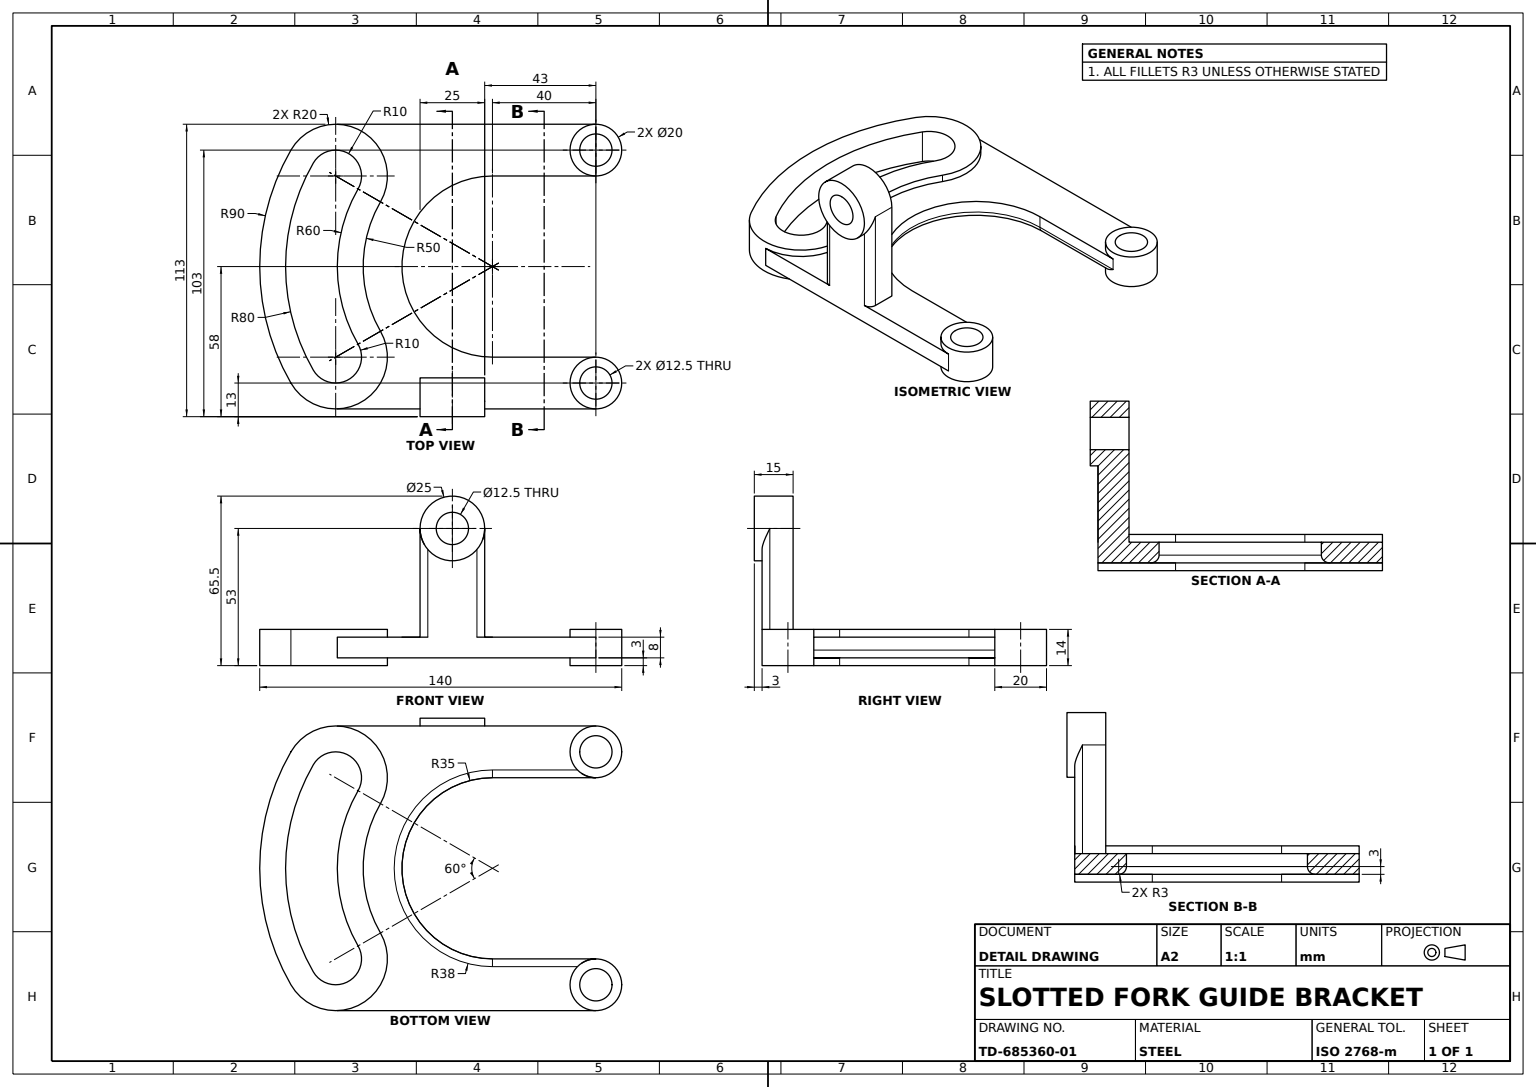
ISO-10303-21;
HEADER;
FILE_DESCRIPTION((''),'2;1');
FILE_NAME('','',(''),(''),'','','');
FILE_SCHEMA(('AUTOMOTIVE_DESIGN'));
ENDSEC;
DATA;
#1=APPLICATION_CONTEXT('');
#2=PRODUCT_CONTEXT('',#1,'mechanical');
#3=PRODUCT('','','',(#2));
#4=PRODUCT_DEFINITION_FORMATION('','',#3);
#5=PRODUCT_DEFINITION_CONTEXT('',#1,'design');
#6=PRODUCT_DEFINITION('','',#4,#5);
#7=PRODUCT_DEFINITION_SHAPE('','',#6);
#8=(LENGTH_UNIT()NAMED_UNIT(*)SI_UNIT(.MILLI.,.METRE.));
#9=(NAMED_UNIT(*)PLANE_ANGLE_UNIT()SI_UNIT($,.RADIAN.));
#10=(NAMED_UNIT(*)SI_UNIT($,.STERADIAN.)SOLID_ANGLE_UNIT());
#11=UNCERTAINTY_MEASURE_WITH_UNIT(LENGTH_MEASURE(0.005),#8,'distance_accuracy_value','');
#12=(GEOMETRIC_REPRESENTATION_CONTEXT(3)GLOBAL_UNCERTAINTY_ASSIGNED_CONTEXT((#11))GLOBAL_UNIT_ASSIGNED_CONTEXT((#8,#9,#10))REPRESENTATION_CONTEXT('',''));
#13=CARTESIAN_POINT('',(-77.942286,-45.,7.));
#14=VERTEX_POINT('',#13);
#15=CARTESIAN_POINT('',(-77.942286,-45.,-7.));
#16=VERTEX_POINT('',#15);
#17=DIRECTION('',(0.,0.,-1.));
#18=VECTOR('',#17,1000.);
#19=LINE('',#13,#18);
#20=EDGE_CURVE('',#14,#16,#19,.T.);
#21=ORIENTED_EDGE('',*,*,#20,.T.);
#22=CARTESIAN_POINT('',(-43.30127,-25.,-7.));
#23=VERTEX_POINT('',#22);
#24=CARTESIAN_POINT('',(-60.621778,-35.,-7.));
#25=DIRECTION('',(0.,0.,1.));
#26=DIRECTION('',(1.,0.,0.));
#27=AXIS2_PLACEMENT_3D('',#24,#25,#26);
#28=CIRCLE('',#27,20.);
#29=EDGE_CURVE('',#16,#23,#28,.T.);
#30=ORIENTED_EDGE('',*,*,#29,.T.);
#31=CARTESIAN_POINT('',(-43.30127,-25.,-4.));
#32=VERTEX_POINT('',#31);
#33=CARTESIAN_POINT('',(-43.30127,-25.,7.));
#34=LINE('',#33,#18);
#35=EDGE_CURVE('',#32,#23,#34,.T.);
#36=ORIENTED_EDGE('',*,*,#35,.F.);
#37=CARTESIAN_POINT('',(-60.,-54.990332,-4.));
#38=VERTEX_POINT('',#37);
#39=CARTESIAN_POINT('',(-60.621778,-35.,-4.));
#40=AXIS2_PLACEMENT_3D('',#39,#25,#26);
#41=CIRCLE('',#40,20.);
#42=EDGE_CURVE('',#32,#38,#41,.F.);
#43=ORIENTED_EDGE('',*,*,#42,.T.);
#44=CARTESIAN_POINT('',(-60.,-54.990332,4.));
#45=VERTEX_POINT('',#44);
#46=CARTESIAN_POINT('',(-60.,-54.990332,7.));
#47=LINE('',#46,#18);
#48=EDGE_CURVE('',#45,#38,#47,.T.);
#49=ORIENTED_EDGE('',*,*,#48,.F.);
#50=CARTESIAN_POINT('',(-43.30127,-25.,4.));
#51=VERTEX_POINT('',#50);
#52=CARTESIAN_POINT('',(-60.621778,-35.,4.));
#53=AXIS2_PLACEMENT_3D('',#52,#25,#26);
#54=CIRCLE('',#53,20.);
#55=EDGE_CURVE('',#51,#45,#54,.F.);
#56=ORIENTED_EDGE('',*,*,#55,.F.);
#57=VERTEX_POINT('',#33);
#58=EDGE_CURVE('',#57,#51,#34,.T.);
#59=ORIENTED_EDGE('',*,*,#58,.F.);
#60=CARTESIAN_POINT('',(-60.621778,-35.,7.));
#61=AXIS2_PLACEMENT_3D('',#60,#25,#26);
#62=CIRCLE('',#61,20.);
#63=EDGE_CURVE('',#14,#57,#62,.T.);
#64=ORIENTED_EDGE('',*,*,#63,.F.);
#65=EDGE_LOOP('',(#21,#30,#36,#43,#49,#56,#59,#64));
#66=FACE_BOUND('',#65,.T.);
#67=DIRECTION('',(-1.,0.,0.));
#68=AXIS2_PLACEMENT_3D('',#60,#17,#67);
#69=CYLINDRICAL_SURFACE('',#68,20.);
#70=ADVANCED_FACE('',(#66),#69,.T.);
#71=CARTESIAN_POINT('',(0.,35.,4.));
#72=VERTEX_POINT('',#71);
#73=CARTESIAN_POINT('',(0.,35.,-1.));
#74=VERTEX_POINT('',#73);
#75=CARTESIAN_POINT('',(0.,35.,-4.));
#76=VECTOR('',#25,1000.);
#77=LINE('',#75,#76);
#78=EDGE_CURVE('',#72,#74,#77,.F.);
#79=ORIENTED_EDGE('',*,*,#78,.F.);
#80=CARTESIAN_POINT('',(0.,-35.,4.));
#81=VERTEX_POINT('',#80);
#82=CARTESIAN_POINT('',(0.,0.,4.));
#83=AXIS2_PLACEMENT_3D('',#82,#17,#26);
#84=CIRCLE('',#83,35.);
#85=EDGE_CURVE('',#72,#81,#84,.F.);
#86=ORIENTED_EDGE('',*,*,#85,.T.);
#87=CARTESIAN_POINT('',(0.,-35.,-1.));
#88=VERTEX_POINT('',#87);
#89=CARTESIAN_POINT('',(0.,-35.,-4.));
#90=LINE('',#89,#76);
#91=EDGE_CURVE('',#81,#88,#90,.F.);
#92=ORIENTED_EDGE('',*,*,#91,.T.);
#93=CARTESIAN_POINT('',(0.,0.,-1.));
#94=AXIS2_PLACEMENT_3D('',#93,#25,#26);
#95=CIRCLE('',#94,35.);
#96=EDGE_CURVE('',#88,#74,#95,.F.);
#97=ORIENTED_EDGE('',*,*,#96,.T.);
#98=EDGE_LOOP('',(#79,#86,#92,#97));
#99=FACE_BOUND('',#98,.T.);
#100=CARTESIAN_POINT('',(0.,0.,-4.));
#101=AXIS2_PLACEMENT_3D('',#100,#25,#26);
#102=CYLINDRICAL_SURFACE('',#101,35.);
#103=ADVANCED_FACE('',(#99),#102,.F.);
#104=CARTESIAN_POINT('',(-25.,-55.,4.));
#105=VERTEX_POINT('',#104);
#106=CARTESIAN_POINT('',(-28.,-52.,4.));
#107=VERTEX_POINT('',#106);
#108=CARTESIAN_POINT('',(-25.,-52.,4.));
#109=AXIS2_PLACEMENT_3D('',#108,#25,#26);
#110=CIRCLE('',#109,3.);
#111=EDGE_CURVE('',#105,#107,#110,.F.);
#112=ORIENTED_EDGE('',*,*,#111,.F.);
#113=CARTESIAN_POINT('',(-25.,-55.,37.875962));
#114=VERTEX_POINT('',#113);
#115=LINE('',#104,#18);
#116=EDGE_CURVE('',#114,#105,#115,.T.);
#117=ORIENTED_EDGE('',*,*,#116,.F.);
#118=CARTESIAN_POINT('',(-28.,-52.,46.));
#119=VERTEX_POINT('',#118);
#120=CARTESIAN_POINT('',(-25.516009,-55.,38.479367));
#121=CARTESIAN_POINT('',(-26.410261,-54.746164,39.758776));
#122=CARTESIAN_POINT('',(-27.646887,-53.736894,42.469166));
#123=CARTESIAN_POINT('',(-28.,-52.688826,44.593938));
#124=B_SPLINE_CURVE_WITH_KNOTS('',3,(#113,#120,#121,#122,#123,#118),.UNSPECIFIED.,.F.,.F.,(4,1,1,4),(0.,0.002348585,0.00469717,0.009394339),.UNSPECIFIED.);
#125=EDGE_CURVE('',#119,#114,#124,.F.);
#126=ORIENTED_EDGE('',*,*,#125,.F.);
#127=LINE('',#118,#18);
#128=EDGE_CURVE('',#107,#119,#127,.F.);
#129=ORIENTED_EDGE('',*,*,#128,.F.);
#130=EDGE_LOOP('',(#112,#117,#126,#129));
#131=FACE_BOUND('',#130,.T.);
#132=CARTESIAN_POINT('',(-25.,-52.,-4.));
#133=AXIS2_PLACEMENT_3D('',#132,#25,#26);
#134=CYLINDRICAL_SURFACE('',#133,3.);
#135=ADVANCED_FACE('',(#131),#134,.T.);
#136=CARTESIAN_POINT('',(50.,45.,7.));
#137=VERTEX_POINT('',#136);
#138=CARTESIAN_POINT('',(40.,45.,7.));
#139=AXIS2_PLACEMENT_3D('',#138,#25,#26);
#140=CIRCLE('',#139,10.);
#141=EDGE_CURVE('',#137,#137,#140,.T.);
#142=ORIENTED_EDGE('',*,*,#141,.F.);
#143=EDGE_LOOP('',(#142));
#144=FACE_BOUND('',#143,.T.);
#145=CARTESIAN_POINT('',(40.,55.,-4.));
#146=VERTEX_POINT('',#145);
#147=CARTESIAN_POINT('',(32.858572,38.,-4.));
#148=VERTEX_POINT('',#147);
#149=CARTESIAN_POINT('',(40.,45.,-4.));
#150=AXIS2_PLACEMENT_3D('',#149,#25,#26);
#151=CIRCLE('',#150,10.);
#152=EDGE_CURVE('',#146,#148,#151,.T.);
#153=ORIENTED_EDGE('',*,*,#152,.F.);
#154=CARTESIAN_POINT('',(40.,55.,4.));
#155=VERTEX_POINT('',#154);
#156=LINE('',#145,#76);
#157=EDGE_CURVE('',#155,#146,#156,.F.);
#158=ORIENTED_EDGE('',*,*,#157,.F.);
#159=CARTESIAN_POINT('',(40.,35.,4.));
#160=VERTEX_POINT('',#159);
#161=CARTESIAN_POINT('',(40.,45.,4.));
#162=AXIS2_PLACEMENT_3D('',#161,#25,#26);
#163=CIRCLE('',#162,10.);
#164=EDGE_CURVE('',#155,#160,#163,.T.);
#165=ORIENTED_EDGE('',*,*,#164,.T.);
#166=CARTESIAN_POINT('',(40.,35.,-1.));
#167=VERTEX_POINT('',#166);
#168=CARTESIAN_POINT('',(40.,35.,-4.));
#169=LINE('',#168,#76);
#170=EDGE_CURVE('',#160,#167,#169,.F.);
#171=ORIENTED_EDGE('',*,*,#170,.T.);
#172=CARTESIAN_POINT('',(33.366096,37.482222,-4.));
#173=CARTESIAN_POINT('',(34.47163,36.581588,-3.74306));
#174=CARTESIAN_POINT('',(36.85864,35.348071,-2.72768));
#175=CARTESIAN_POINT('',(38.746946,35.,-1.686325));
#176=B_SPLINE_CURVE_WITH_KNOTS('',3,(#147,#172,#173,#174,#175,#166),.UNSPECIFIED.,.F.,.F.,(4,1,1,4),(0.,0.002143051,0.004286102,0.008572205),.UNSPECIFIED.);
#177=EDGE_CURVE('',#167,#148,#176,.F.);
#178=ORIENTED_EDGE('',*,*,#177,.T.);
#179=EDGE_LOOP('',(#153,#158,#165,#171,#178));
#180=FACE_BOUND('',#179,.T.);
#181=CARTESIAN_POINT('',(50.,45.,-7.));
#182=VERTEX_POINT('',#181);
#183=CARTESIAN_POINT('',(40.,45.,-7.));
#184=AXIS2_PLACEMENT_3D('',#183,#25,#26);
#185=CIRCLE('',#184,10.);
#186=EDGE_CURVE('',#182,#182,#185,.T.);
#187=ORIENTED_EDGE('',*,*,#186,.T.);
#188=EDGE_LOOP('',(#187));
#189=FACE_BOUND('',#188,.T.);
#190=CYLINDRICAL_SURFACE('',#150,10.);
#191=ADVANCED_FACE('',(#144,#180,#189),#190,.T.);
#192=CARTESIAN_POINT('',(50.,-45.,-7.));
#193=VERTEX_POINT('',#192);
#194=CARTESIAN_POINT('',(40.,-45.,-7.));
#195=AXIS2_PLACEMENT_3D('',#194,#17,#26);
#196=CIRCLE('',#195,10.);
#197=EDGE_CURVE('',#193,#193,#196,.T.);
#198=ORIENTED_EDGE('',*,*,#197,.F.);
#199=EDGE_LOOP('',(#198));
#200=FACE_BOUND('',#199,.T.);
#201=CARTESIAN_POINT('',(50.,-45.,7.));
#202=VERTEX_POINT('',#201);
#203=CARTESIAN_POINT('',(40.,-45.,7.));
#204=AXIS2_PLACEMENT_3D('',#203,#17,#26);
#205=CIRCLE('',#204,10.);
#206=EDGE_CURVE('',#202,#202,#205,.T.);
#207=ORIENTED_EDGE('',*,*,#206,.T.);
#208=EDGE_LOOP('',(#207));
#209=FACE_BOUND('',#208,.T.);
#210=CARTESIAN_POINT('',(40.,-35.,4.));
#211=VERTEX_POINT('',#210);
#212=CARTESIAN_POINT('',(40.,-55.,4.));
#213=VERTEX_POINT('',#212);
#214=CARTESIAN_POINT('',(40.,-45.,4.));
#215=AXIS2_PLACEMENT_3D('',#214,#25,#26);
#216=CIRCLE('',#215,10.);
#217=EDGE_CURVE('',#211,#213,#216,.T.);
#218=ORIENTED_EDGE('',*,*,#217,.T.);
#219=CARTESIAN_POINT('',(40.,-55.,-4.));
#220=VERTEX_POINT('',#219);
#221=LINE('',#219,#76);
#222=EDGE_CURVE('',#213,#220,#221,.F.);
#223=ORIENTED_EDGE('',*,*,#222,.T.);
#224=CARTESIAN_POINT('',(32.858572,-38.,-4.));
#225=VERTEX_POINT('',#224);
#226=CARTESIAN_POINT('',(40.,-45.,-4.));
#227=AXIS2_PLACEMENT_3D('',#226,#25,#26);
#228=CIRCLE('',#227,10.);
#229=EDGE_CURVE('',#225,#220,#228,.T.);
#230=ORIENTED_EDGE('',*,*,#229,.F.);
#231=CARTESIAN_POINT('',(40.,-35.,-1.));
#232=VERTEX_POINT('',#231);
#233=CARTESIAN_POINT('',(33.366096,-37.482222,-4.));
#234=CARTESIAN_POINT('',(34.47163,-36.581588,-3.74306));
#235=CARTESIAN_POINT('',(36.85864,-35.348071,-2.72768));
#236=CARTESIAN_POINT('',(38.746946,-35.,-1.686325));
#237=B_SPLINE_CURVE_WITH_KNOTS('',3,(#224,#233,#234,#235,#236,#231),.UNSPECIFIED.,.F.,.F.,(4,1,1,4),(0.,0.002143051,0.004286102,0.008572205),.UNSPECIFIED.);
#238=EDGE_CURVE('',#225,#232,#237,.T.);
#239=ORIENTED_EDGE('',*,*,#238,.T.);
#240=CARTESIAN_POINT('',(40.,-35.,-4.));
#241=LINE('',#240,#76);
#242=EDGE_CURVE('',#211,#232,#241,.F.);
#243=ORIENTED_EDGE('',*,*,#242,.F.);
#244=EDGE_LOOP('',(#218,#223,#230,#239,#243));
#245=FACE_BOUND('',#244,.T.);
#246=CYLINDRICAL_SURFACE('',#227,10.);
#247=ADVANCED_FACE('',(#200,#209,#245),#246,.T.);
#248=CARTESIAN_POINT('',(-43.30127,25.,-4.));
#249=VERTEX_POINT('',#248);
#250=CIRCLE('',#101,50.);
#251=EDGE_CURVE('',#249,#32,#250,.T.);
#252=ORIENTED_EDGE('',*,*,#251,.F.);
#253=CARTESIAN_POINT('',(-60.,54.990332,-4.));
#254=VERTEX_POINT('',#253);
#255=CARTESIAN_POINT('',(-60.621778,35.,-4.));
#256=AXIS2_PLACEMENT_3D('',#255,#25,#26);
#257=CIRCLE('',#256,20.);
#258=EDGE_CURVE('',#254,#249,#257,.F.);
#259=ORIENTED_EDGE('',*,*,#258,.F.);
#260=CARTESIAN_POINT('',(-60.,55.,-4.));
#261=VERTEX_POINT('',#260);
#262=DIRECTION('',(0.,-1.,0.));
#263=VECTOR('',#262,1000.);
#264=LINE('',#260,#263);
#265=EDGE_CURVE('',#254,#261,#264,.F.);
#266=ORIENTED_EDGE('',*,*,#265,.T.);
#267=VECTOR('',#67,1000.);
#268=LINE('',#145,#267);
#269=EDGE_CURVE('',#261,#146,#268,.F.);
#270=ORIENTED_EDGE('',*,*,#269,.T.);
#271=ORIENTED_EDGE('',*,*,#152,.T.);
#272=CARTESIAN_POINT('',(0.,38.,-4.));
#273=VERTEX_POINT('',#272);
#274=LINE('',#272,#267);
#275=EDGE_CURVE('',#148,#273,#274,.T.);
#276=ORIENTED_EDGE('',*,*,#275,.T.);
#277=CARTESIAN_POINT('',(0.,-38.,-4.));
#278=VERTEX_POINT('',#277);
#279=CIRCLE('',#101,38.);
#280=EDGE_CURVE('',#273,#278,#279,.T.);
#281=ORIENTED_EDGE('',*,*,#280,.T.);
#282=CARTESIAN_POINT('',(40.,-38.,-4.));
#283=VECTOR('',#26,1000.);
#284=LINE('',#282,#283);
#285=EDGE_CURVE('',#278,#225,#284,.T.);
#286=ORIENTED_EDGE('',*,*,#285,.T.);
#287=ORIENTED_EDGE('',*,*,#229,.T.);
#288=CARTESIAN_POINT('',(-60.,-55.,-4.));
#289=VERTEX_POINT('',#288);
#290=LINE('',#288,#283);
#291=EDGE_CURVE('',#220,#289,#290,.F.);
#292=ORIENTED_EDGE('',*,*,#291,.T.);
#293=EDGE_CURVE('',#289,#38,#264,.F.);
#294=ORIENTED_EDGE('',*,*,#293,.T.);
#295=ORIENTED_EDGE('',*,*,#42,.F.);
#296=EDGE_LOOP('',(#252,#259,#266,#270,#271,#276,#281,#286,#287,#292,#294,#295));
#297=FACE_BOUND('',#296,.T.);
#298=PLANE('',#227);
#299=ADVANCED_FACE('',(#297),#298,.F.);
#300=CARTESIAN_POINT('',(-60.,54.990332,4.));
#301=VERTEX_POINT('',#300);
#302=CARTESIAN_POINT('',(-60.,55.,4.));
#303=VERTEX_POINT('',#302);
#304=LINE('',#302,#263);
#305=EDGE_CURVE('',#301,#303,#304,.F.);
#306=ORIENTED_EDGE('',*,*,#305,.F.);
#307=CARTESIAN_POINT('',(-43.30127,25.,4.));
#308=VERTEX_POINT('',#307);
#309=CARTESIAN_POINT('',(-60.621778,35.,4.));
#310=AXIS2_PLACEMENT_3D('',#309,#25,#26);
#311=CIRCLE('',#310,20.);
#312=EDGE_CURVE('',#301,#308,#311,.F.);
#313=ORIENTED_EDGE('',*,*,#312,.T.);
#314=AXIS2_PLACEMENT_3D('',#82,#25,#26);
#315=CIRCLE('',#314,50.);
#316=EDGE_CURVE('',#308,#51,#315,.T.);
#317=ORIENTED_EDGE('',*,*,#316,.T.);
#318=ORIENTED_EDGE('',*,*,#55,.T.);
#319=CARTESIAN_POINT('',(-60.,-55.,4.));
#320=VERTEX_POINT('',#319);
#321=EDGE_CURVE('',#320,#45,#304,.F.);
#322=ORIENTED_EDGE('',*,*,#321,.F.);
#323=LINE('',#319,#283);
#324=EDGE_CURVE('',#105,#320,#323,.F.);
#325=ORIENTED_EDGE('',*,*,#324,.F.);
#326=ORIENTED_EDGE('',*,*,#111,.T.);
#327=CARTESIAN_POINT('',(-28.,-43.,4.));
#328=VERTEX_POINT('',#327);
#329=CARTESIAN_POINT('',(-28.,-45.,4.));
#330=DIRECTION('',(0.,1.,0.));
#331=VECTOR('',#330,1000.);
#332=LINE('',#329,#331);
#333=EDGE_CURVE('',#107,#328,#332,.T.);
#334=ORIENTED_EDGE('',*,*,#333,.T.);
#335=CARTESIAN_POINT('',(-3.,-43.,4.));
#336=VERTEX_POINT('',#335);
#337=CARTESIAN_POINT('',(40.,-43.,4.));
#338=LINE('',#337,#283);
#339=EDGE_CURVE('',#328,#336,#338,.T.);
#340=ORIENTED_EDGE('',*,*,#339,.T.);
#341=CARTESIAN_POINT('',(-3.,-52.,4.));
#342=VERTEX_POINT('',#341);
#343=CARTESIAN_POINT('',(-3.,-45.,4.));
#344=LINE('',#343,#263);
#345=EDGE_CURVE('',#336,#342,#344,.T.);
#346=ORIENTED_EDGE('',*,*,#345,.T.);
#347=CARTESIAN_POINT('',(-6.,-55.,4.));
#348=VERTEX_POINT('',#347);
#349=CARTESIAN_POINT('',(-6.,-52.,4.));
#350=AXIS2_PLACEMENT_3D('',#349,#25,#26);
#351=CIRCLE('',#350,3.);
#352=EDGE_CURVE('',#342,#348,#351,.F.);
#353=ORIENTED_EDGE('',*,*,#352,.T.);
#354=EDGE_CURVE('',#213,#348,#323,.F.);
#355=ORIENTED_EDGE('',*,*,#354,.F.);
#356=ORIENTED_EDGE('',*,*,#217,.F.);
#357=LINE('',#210,#267);
#358=EDGE_CURVE('',#81,#211,#357,.F.);
#359=ORIENTED_EDGE('',*,*,#358,.F.);
#360=ORIENTED_EDGE('',*,*,#85,.F.);
#361=LINE('',#71,#283);
#362=EDGE_CURVE('',#160,#72,#361,.F.);
#363=ORIENTED_EDGE('',*,*,#362,.F.);
#364=ORIENTED_EDGE('',*,*,#164,.F.);
#365=LINE('',#154,#267);
#366=EDGE_CURVE('',#303,#155,#365,.F.);
#367=ORIENTED_EDGE('',*,*,#366,.F.);
#368=EDGE_LOOP('',(#306,#313,#317,#318,#322,#325,#326,#334,#340,#346,#353,#355,#356,#359,#360,#363,#364,#367));
#369=FACE_BOUND('',#368,.T.);
#370=PLANE('',#215);
#371=ADVANCED_FACE('',(#369),#370,.T.);
#372=CARTESIAN_POINT('',(-43.30127,25.,-7.));
#373=VERTEX_POINT('',#372);
#374=CARTESIAN_POINT('',(-43.30127,25.,7.));
#375=LINE('',#374,#18);
#376=EDGE_CURVE('',#249,#373,#375,.T.);
#377=ORIENTED_EDGE('',*,*,#376,.F.);
#378=ORIENTED_EDGE('',*,*,#251,.T.);
#379=ORIENTED_EDGE('',*,*,#35,.T.);
#380=CARTESIAN_POINT('',(0.,0.,-7.));
#381=AXIS2_PLACEMENT_3D('',#380,#17,#26);
#382=CIRCLE('',#381,50.);
#383=EDGE_CURVE('',#23,#373,#382,.T.);
#384=ORIENTED_EDGE('',*,*,#383,.T.);
#385=EDGE_LOOP('',(#377,#378,#379,#384));
#386=FACE_BOUND('',#385,.T.);
#387=CARTESIAN_POINT('',(0.,0.,7.));
#388=AXIS2_PLACEMENT_3D('',#387,#17,#67);
#389=CYLINDRICAL_SURFACE('',#388,50.);
#390=ADVANCED_FACE('',(#386),#389,.F.);
#391=CARTESIAN_POINT('',(-6.,-55.,37.875962));
#392=VERTEX_POINT('',#391);
#393=CARTESIAN_POINT('',(-15.5,-55.,46.));
#394=AXIS2_PLACEMENT_3D('',#393,#262,#17);
#395=CIRCLE('',#394,12.5);
#396=EDGE_CURVE('',#392,#114,#395,.F.);
#397=ORIENTED_EDGE('',*,*,#396,.F.);
#398=CARTESIAN_POINT('',(-3.,-52.,46.));
#399=VERTEX_POINT('',#398);
#400=CARTESIAN_POINT('',(-5.483991,-55.,38.479367));
#401=CARTESIAN_POINT('',(-4.589739,-54.746164,39.758776));
#402=CARTESIAN_POINT('',(-3.353113,-53.736894,42.469166));
#403=CARTESIAN_POINT('',(-3.,-52.688826,44.593938));
#404=B_SPLINE_CURVE_WITH_KNOTS('',3,(#391,#400,#401,#402,#403,#398),.UNSPECIFIED.,.F.,.F.,(4,1,1,4),(0.,0.002348585,0.00469717,0.009394339),.UNSPECIFIED.);
#405=EDGE_CURVE('',#392,#399,#404,.T.);
#406=ORIENTED_EDGE('',*,*,#405,.T.);
#407=CARTESIAN_POINT('',(-3.,-43.,46.));
#408=VERTEX_POINT('',#407);
#409=CARTESIAN_POINT('',(-3.,-55.,46.));
#410=LINE('',#409,#331);
#411=EDGE_CURVE('',#399,#408,#410,.T.);
#412=ORIENTED_EDGE('',*,*,#411,.T.);
#413=CARTESIAN_POINT('',(-28.,-43.,46.));
#414=VERTEX_POINT('',#413);
#415=CARTESIAN_POINT('',(-15.5,-43.,46.));
#416=AXIS2_PLACEMENT_3D('',#415,#262,#26);
#417=CIRCLE('',#416,12.5);
#418=EDGE_CURVE('',#408,#414,#417,.T.);
#419=ORIENTED_EDGE('',*,*,#418,.T.);
#420=CARTESIAN_POINT('',(-28.,-55.,46.));
#421=LINE('',#420,#331);
#422=EDGE_CURVE('',#119,#414,#421,.T.);
#423=ORIENTED_EDGE('',*,*,#422,.F.);
#424=ORIENTED_EDGE('',*,*,#125,.T.);
#425=EDGE_LOOP('',(#397,#406,#412,#419,#423,#424));
#426=FACE_BOUND('',#425,.T.);
#427=CARTESIAN_POINT('',(-3.,-58.,46.));
#428=VERTEX_POINT('',#427);
#429=CARTESIAN_POINT('',(-15.5,-58.,46.));
#430=AXIS2_PLACEMENT_3D('',#429,#262,#26);
#431=CIRCLE('',#430,12.5);
#432=EDGE_CURVE('',#428,#428,#431,.T.);
#433=ORIENTED_EDGE('',*,*,#432,.F.);
#434=EDGE_LOOP('',(#433));
#435=FACE_BOUND('',#434,.T.);
#436=AXIS2_PLACEMENT_3D('',#429,#330,#25);
#437=CYLINDRICAL_SURFACE('',#436,12.5);
#438=ADVANCED_FACE('',(#426,#435),#437,.T.);
#439=CARTESIAN_POINT('',(46.25,45.,-7.));
#440=VERTEX_POINT('',#439);
#441=CIRCLE('',#184,6.25);
#442=EDGE_CURVE('',#440,#440,#441,.T.);
#443=ORIENTED_EDGE('',*,*,#442,.F.);
#444=EDGE_LOOP('',(#443));
#445=FACE_BOUND('',#444,.T.);
#446=CARTESIAN_POINT('',(33.75,45.,7.));
#447=VERTEX_POINT('',#446);
#448=AXIS2_PLACEMENT_3D('',#138,#17,#67);
#449=CIRCLE('',#448,6.25);
#450=EDGE_CURVE('',#447,#447,#449,.T.);
#451=ORIENTED_EDGE('',*,*,#450,.F.);
#452=EDGE_LOOP('',(#451));
#453=FACE_BOUND('',#452,.T.);
#454=CYLINDRICAL_SURFACE('',#448,6.25);
#455=ADVANCED_FACE('',(#445,#453),#454,.F.);
#456=ORIENTED_EDGE('',*,*,#20,.F.);
#457=CARTESIAN_POINT('',(-77.942286,45.,7.));
#458=VERTEX_POINT('',#457);
#459=AXIS2_PLACEMENT_3D('',#387,#25,#26);
#460=CIRCLE('',#459,90.);
#461=EDGE_CURVE('',#458,#14,#460,.T.);
#462=ORIENTED_EDGE('',*,*,#461,.F.);
#463=CARTESIAN_POINT('',(-77.942286,45.,-7.));
#464=VERTEX_POINT('',#463);
#465=LINE('',#457,#18);
#466=EDGE_CURVE('',#458,#464,#465,.T.);
#467=ORIENTED_EDGE('',*,*,#466,.T.);
#468=AXIS2_PLACEMENT_3D('',#380,#25,#26);
#469=CIRCLE('',#468,90.);
#470=EDGE_CURVE('',#464,#16,#469,.T.);
#471=ORIENTED_EDGE('',*,*,#470,.T.);
#472=EDGE_LOOP('',(#456,#462,#467,#471));
#473=FACE_BOUND('',#472,.T.);
#474=CYLINDRICAL_SURFACE('',#388,90.);
#475=ADVANCED_FACE('',(#473),#474,.T.);
#476=ORIENTED_EDGE('',*,*,#258,.T.);
#477=ORIENTED_EDGE('',*,*,#376,.T.);
#478=CARTESIAN_POINT('',(-60.621778,35.,-7.));
#479=AXIS2_PLACEMENT_3D('',#478,#25,#26);
#480=CIRCLE('',#479,20.);
#481=EDGE_CURVE('',#373,#464,#480,.T.);
#482=ORIENTED_EDGE('',*,*,#481,.T.);
#483=ORIENTED_EDGE('',*,*,#466,.F.);
#484=VERTEX_POINT('',#374);
#485=CARTESIAN_POINT('',(-60.621778,35.,7.));
#486=AXIS2_PLACEMENT_3D('',#485,#25,#26);
#487=CIRCLE('',#486,20.);
#488=EDGE_CURVE('',#484,#458,#487,.T.);
#489=ORIENTED_EDGE('',*,*,#488,.F.);
#490=EDGE_CURVE('',#484,#308,#375,.T.);
#491=ORIENTED_EDGE('',*,*,#490,.T.);
#492=ORIENTED_EDGE('',*,*,#312,.F.);
#493=CARTESIAN_POINT('',(-60.,54.990332,7.));
#494=LINE('',#493,#18);
#495=EDGE_CURVE('',#254,#301,#494,.F.);
#496=ORIENTED_EDGE('',*,*,#495,.F.);
#497=EDGE_LOOP('',(#476,#477,#482,#483,#489,#491,#492,#496));
#498=FACE_BOUND('',#497,.T.);
#499=AXIS2_PLACEMENT_3D('',#485,#17,#67);
#500=CYLINDRICAL_SURFACE('',#499,20.);
#501=ADVANCED_FACE('',(#498),#500,.T.);
#502=LINE('',#260,#76);
#503=EDGE_CURVE('',#303,#261,#502,.F.);
#504=ORIENTED_EDGE('',*,*,#503,.T.);
#505=ORIENTED_EDGE('',*,*,#265,.F.);
#506=ORIENTED_EDGE('',*,*,#495,.T.);
#507=ORIENTED_EDGE('',*,*,#305,.T.);
#508=EDGE_LOOP('',(#504,#505,#506,#507));
#509=FACE_BOUND('',#508,.T.);
#510=AXIS2_PLACEMENT_3D('',#260,#67,#25);
#511=PLANE('',#510);
#512=ADVANCED_FACE('',(#509),#511,.T.);
#513=CARTESIAN_POINT('',(-69.282032,40.,7.));
#514=VERTEX_POINT('',#513);
#515=CARTESIAN_POINT('',(-69.282032,-40.,7.));
#516=VERTEX_POINT('',#515);
#517=CIRCLE('',#459,80.);
#518=EDGE_CURVE('',#514,#516,#517,.T.);
#519=ORIENTED_EDGE('',*,*,#518,.T.);
#520=CARTESIAN_POINT('',(-69.282032,-40.,-7.));
#521=VERTEX_POINT('',#520);
#522=LINE('',#515,#18);
#523=EDGE_CURVE('',#516,#521,#522,.T.);
#524=ORIENTED_EDGE('',*,*,#523,.T.);
#525=CARTESIAN_POINT('',(-69.282032,40.,-7.));
#526=VERTEX_POINT('',#525);
#527=CIRCLE('',#468,80.);
#528=EDGE_CURVE('',#526,#521,#527,.T.);
#529=ORIENTED_EDGE('',*,*,#528,.F.);
#530=LINE('',#513,#18);
#531=EDGE_CURVE('',#514,#526,#530,.T.);
#532=ORIENTED_EDGE('',*,*,#531,.F.);
#533=EDGE_LOOP('',(#519,#524,#529,#532));
#534=FACE_BOUND('',#533,.T.);
#535=CYLINDRICAL_SURFACE('',#388,80.);
#536=ADVANCED_FACE('',(#534),#535,.F.);
#537=ORIENTED_EDGE('',*,*,#78,.T.);
#538=LINE('',#166,#267);
#539=EDGE_CURVE('',#74,#167,#538,.F.);
#540=ORIENTED_EDGE('',*,*,#539,.T.);
#541=ORIENTED_EDGE('',*,*,#170,.F.);
#542=ORIENTED_EDGE('',*,*,#362,.T.);
#543=EDGE_LOOP('',(#537,#540,#541,#542));
#544=FACE_BOUND('',#543,.T.);
#545=AXIS2_PLACEMENT_3D('',#75,#262,#17);
#546=PLANE('',#545);
#547=ADVANCED_FACE('',(#544),#546,.T.);
#548=CARTESIAN_POINT('',(33.75,-45.,7.));
#549=VERTEX_POINT('',#548);
#550=AXIS2_PLACEMENT_3D('',#203,#17,#67);
#551=CIRCLE('',#550,6.25);
#552=EDGE_CURVE('',#549,#549,#551,.T.);
#553=ORIENTED_EDGE('',*,*,#552,.F.);
#554=EDGE_LOOP('',(#553));
#555=FACE_BOUND('',#554,.T.);
#556=CARTESIAN_POINT('',(33.75,-45.,-7.));
#557=VERTEX_POINT('',#556);
#558=AXIS2_PLACEMENT_3D('',#194,#17,#67);
#559=CIRCLE('',#558,6.25);
#560=EDGE_CURVE('',#557,#557,#559,.T.);
#561=ORIENTED_EDGE('',*,*,#560,.T.);
#562=EDGE_LOOP('',(#561));
#563=FACE_BOUND('',#562,.T.);
#564=CYLINDRICAL_SURFACE('',#550,6.25);
#565=ADVANCED_FACE('',(#555,#563),#564,.F.);
#566=ORIENTED_EDGE('',*,*,#503,.F.);
#567=ORIENTED_EDGE('',*,*,#366,.T.);
#568=ORIENTED_EDGE('',*,*,#157,.T.);
#569=ORIENTED_EDGE('',*,*,#269,.F.);
#570=EDGE_LOOP('',(#566,#567,#568,#569));
#571=FACE_BOUND('',#570,.T.);
#572=AXIS2_PLACEMENT_3D('',#145,#330,#25);
#573=PLANE('',#572);
#574=ADVANCED_FACE('',(#571),#573,.T.);
#575=ORIENTED_EDGE('',*,*,#358,.T.);
#576=ORIENTED_EDGE('',*,*,#242,.T.);
#577=LINE('',#87,#283);
#578=EDGE_CURVE('',#232,#88,#577,.F.);
#579=ORIENTED_EDGE('',*,*,#578,.T.);
#580=ORIENTED_EDGE('',*,*,#91,.F.);
#581=EDGE_LOOP('',(#575,#576,#579,#580));
#582=FACE_BOUND('',#581,.T.);
#583=AXIS2_PLACEMENT_3D('',#240,#330,#25);
#584=PLANE('',#583);
#585=ADVANCED_FACE('',(#582),#584,.T.);
#586=ORIENTED_EDGE('',*,*,#280,.F.);
#587=CARTESIAN_POINT('',(0.,38.,-1.));
#588=AXIS2_PLACEMENT_3D('',#587,#26,#17);
#589=CIRCLE('',#588,3.);
#590=EDGE_CURVE('',#74,#273,#589,.T.);
#591=ORIENTED_EDGE('',*,*,#590,.F.);
#592=ORIENTED_EDGE('',*,*,#96,.F.);
#593=CARTESIAN_POINT('',(0.,-38.,-1.));
#594=AXIS2_PLACEMENT_3D('',#593,#67,#25);
#595=CIRCLE('',#594,3.);
#596=EDGE_CURVE('',#88,#278,#595,.T.);
#597=ORIENTED_EDGE('',*,*,#596,.T.);
#598=EDGE_LOOP('',(#586,#591,#592,#597));
#599=FACE_BOUND('',#598,.T.);
#600=TOROIDAL_SURFACE('',#94,38.,3.);
#601=ADVANCED_FACE('',(#599),#600,.T.);
#602=ORIENTED_EDGE('',*,*,#238,.F.);
#603=ORIENTED_EDGE('',*,*,#285,.F.);
#604=ORIENTED_EDGE('',*,*,#596,.F.);
#605=ORIENTED_EDGE('',*,*,#578,.F.);
#606=EDGE_LOOP('',(#602,#603,#604,#605));
#607=FACE_BOUND('',#606,.T.);
#608=CARTESIAN_POINT('',(40.,-38.,-1.));
#609=AXIS2_PLACEMENT_3D('',#608,#67,#25);
#610=CYLINDRICAL_SURFACE('',#609,3.);
#611=ADVANCED_FACE('',(#607),#610,.T.);
#612=CARTESIAN_POINT('',(-15.5,-43.,39.75));
#613=VERTEX_POINT('',#612);
#614=AXIS2_PLACEMENT_3D('',#415,#262,#17);
#615=CIRCLE('',#614,6.25);
#616=EDGE_CURVE('',#613,#613,#615,.T.);
#617=ORIENTED_EDGE('',*,*,#616,.T.);
#618=EDGE_LOOP('',(#617));
#619=FACE_BOUND('',#618,.T.);
#620=LINE('',#413,#18);
#621=EDGE_CURVE('',#414,#328,#620,.T.);
#622=ORIENTED_EDGE('',*,*,#621,.F.);
#623=ORIENTED_EDGE('',*,*,#418,.F.);
#624=CARTESIAN_POINT('',(-3.,-43.,0.));
#625=LINE('',#624,#76);
#626=EDGE_CURVE('',#336,#408,#625,.T.);
#627=ORIENTED_EDGE('',*,*,#626,.F.);
#628=ORIENTED_EDGE('',*,*,#339,.F.);
#629=EDGE_LOOP('',(#622,#623,#627,#628));
#630=FACE_BOUND('',#629,.T.);
#631=CARTESIAN_POINT('',(0.,-43.,0.));
#632=AXIS2_PLACEMENT_3D('',#631,#262,#17);
#633=PLANE('',#632);
#634=ADVANCED_FACE('',(#619,#630),#633,.F.);
#635=ORIENTED_EDGE('',*,*,#275,.F.);
#636=ORIENTED_EDGE('',*,*,#177,.F.);
#637=ORIENTED_EDGE('',*,*,#539,.F.);
#638=ORIENTED_EDGE('',*,*,#590,.T.);
#639=EDGE_LOOP('',(#635,#636,#637,#638));
#640=FACE_BOUND('',#639,.T.);
#641=CARTESIAN_POINT('',(40.,38.,-1.));
#642=AXIS2_PLACEMENT_3D('',#641,#26,#17);
#643=CYLINDRICAL_SURFACE('',#642,3.);
#644=ADVANCED_FACE('',(#640),#643,.T.);
#645=CARTESIAN_POINT('',(-51.961524,30.,7.));
#646=VERTEX_POINT('',#645);
#647=CARTESIAN_POINT('',(-51.961524,30.,-7.));
#648=VERTEX_POINT('',#647);
#649=LINE('',#645,#18);
#650=EDGE_CURVE('',#646,#648,#649,.T.);
#651=ORIENTED_EDGE('',*,*,#650,.T.);
#652=CARTESIAN_POINT('',(-51.961524,-30.,-7.));
#653=VERTEX_POINT('',#652);
#654=CIRCLE('',#381,60.);
#655=EDGE_CURVE('',#653,#648,#654,.T.);
#656=ORIENTED_EDGE('',*,*,#655,.F.);
#657=CARTESIAN_POINT('',(-51.961524,-30.,7.));
#658=VERTEX_POINT('',#657);
#659=LINE('',#657,#18);
#660=EDGE_CURVE('',#658,#653,#659,.T.);
#661=ORIENTED_EDGE('',*,*,#660,.F.);
#662=AXIS2_PLACEMENT_3D('',#387,#17,#26);
#663=CIRCLE('',#662,60.);
#664=EDGE_CURVE('',#658,#646,#663,.T.);
#665=ORIENTED_EDGE('',*,*,#664,.T.);
#666=EDGE_LOOP('',(#651,#656,#661,#665));
#667=FACE_BOUND('',#666,.T.);
#668=CYLINDRICAL_SURFACE('',#388,60.);
#669=ADVANCED_FACE('',(#667),#668,.T.);
#670=ORIENTED_EDGE('',*,*,#141,.T.);
#671=EDGE_LOOP('',(#670));
#672=FACE_BOUND('',#671,.T.);
#673=ORIENTED_EDGE('',*,*,#450,.T.);
#674=EDGE_LOOP('',(#673));
#675=FACE_BOUND('',#674,.T.);
#676=PLANE('',#139);
#677=ADVANCED_FACE('',(#672,#675),#676,.T.);
#678=ORIENTED_EDGE('',*,*,#442,.T.);
#679=EDGE_LOOP('',(#678));
#680=FACE_BOUND('',#679,.T.);
#681=ORIENTED_EDGE('',*,*,#186,.F.);
#682=EDGE_LOOP('',(#681));
#683=FACE_BOUND('',#682,.T.);
#684=PLANE('',#184);
#685=ADVANCED_FACE('',(#680,#683),#684,.F.);
#686=CARTESIAN_POINT('',(-15.5,-58.,52.25));
#687=VERTEX_POINT('',#686);
#688=CIRCLE('',#436,6.25);
#689=EDGE_CURVE('',#687,#687,#688,.T.);
#690=ORIENTED_EDGE('',*,*,#689,.F.);
#691=EDGE_LOOP('',(#690));
#692=FACE_BOUND('',#691,.T.);
#693=ORIENTED_EDGE('',*,*,#616,.F.);
#694=EDGE_LOOP('',(#693));
#695=FACE_BOUND('',#694,.T.);
#696=CYLINDRICAL_SURFACE('',#436,6.25);
#697=ADVANCED_FACE('',(#692,#695),#696,.F.);
#698=ORIENTED_EDGE('',*,*,#128,.T.);
#699=ORIENTED_EDGE('',*,*,#422,.T.);
#700=ORIENTED_EDGE('',*,*,#621,.T.);
#701=ORIENTED_EDGE('',*,*,#333,.F.);
#702=EDGE_LOOP('',(#698,#699,#700,#701));
#703=FACE_BOUND('',#702,.T.);
#704=AXIS2_PLACEMENT_3D('',#420,#26,#17);
#705=PLANE('',#704);
#706=ADVANCED_FACE('',(#703),#705,.F.);
#707=LINE('',#288,#76);
#708=EDGE_CURVE('',#320,#289,#707,.F.);
#709=ORIENTED_EDGE('',*,*,#708,.T.);
#710=ORIENTED_EDGE('',*,*,#291,.F.);
#711=ORIENTED_EDGE('',*,*,#222,.F.);
#712=ORIENTED_EDGE('',*,*,#354,.T.);
#713=CARTESIAN_POINT('',(-6.,-55.,46.));
#714=LINE('',#713,#76);
#715=EDGE_CURVE('',#348,#392,#714,.T.);
#716=ORIENTED_EDGE('',*,*,#715,.T.);
#717=ORIENTED_EDGE('',*,*,#396,.T.);
#718=ORIENTED_EDGE('',*,*,#116,.T.);
#719=ORIENTED_EDGE('',*,*,#324,.T.);
#720=EDGE_LOOP('',(#709,#710,#711,#712,#716,#717,#718,#719));
#721=FACE_BOUND('',#720,.T.);
#722=AXIS2_PLACEMENT_3D('',#288,#262,#17);
#723=PLANE('',#722);
#724=ADVANCED_FACE('',(#721),#723,.T.);
#725=ORIENTED_EDGE('',*,*,#708,.F.);
#726=ORIENTED_EDGE('',*,*,#321,.T.);
#727=ORIENTED_EDGE('',*,*,#48,.T.);
#728=ORIENTED_EDGE('',*,*,#293,.F.);
#729=EDGE_LOOP('',(#725,#726,#727,#728));
#730=FACE_BOUND('',#729,.T.);
#731=ADVANCED_FACE('',(#730),#511,.T.);
#732=ORIENTED_EDGE('',*,*,#29,.F.);
#733=ORIENTED_EDGE('',*,*,#470,.F.);
#734=ORIENTED_EDGE('',*,*,#481,.F.);
#735=ORIENTED_EDGE('',*,*,#383,.F.);
#736=EDGE_LOOP('',(#732,#733,#734,#735));
#737=FACE_BOUND('',#736,.T.);
#738=ORIENTED_EDGE('',*,*,#528,.T.);
#739=CIRCLE('',#27,10.);
#740=EDGE_CURVE('',#521,#653,#739,.T.);
#741=ORIENTED_EDGE('',*,*,#740,.T.);
#742=ORIENTED_EDGE('',*,*,#655,.T.);
#743=CIRCLE('',#479,10.);
#744=EDGE_CURVE('',#648,#526,#743,.T.);
#745=ORIENTED_EDGE('',*,*,#744,.T.);
#746=EDGE_LOOP('',(#738,#741,#742,#745));
#747=FACE_BOUND('',#746,.T.);
#748=CARTESIAN_POINT('',(-30.310889,-17.5,-7.));
#749=AXIS2_PLACEMENT_3D('',#748,#25,#26);
#750=PLANE('',#749);
#751=ADVANCED_FACE('',(#737,#747),#750,.F.);
#752=ORIENTED_EDGE('',*,*,#531,.T.);
#753=ORIENTED_EDGE('',*,*,#744,.F.);
#754=ORIENTED_EDGE('',*,*,#650,.F.);
#755=CIRCLE('',#486,10.);
#756=EDGE_CURVE('',#646,#514,#755,.T.);
#757=ORIENTED_EDGE('',*,*,#756,.T.);
#758=EDGE_LOOP('',(#752,#753,#754,#757));
#759=FACE_BOUND('',#758,.T.);
#760=CYLINDRICAL_SURFACE('',#499,10.);
#761=ADVANCED_FACE('',(#759),#760,.F.);
#762=ORIENTED_EDGE('',*,*,#197,.T.);
#763=EDGE_LOOP('',(#762));
#764=FACE_BOUND('',#763,.T.);
#765=ORIENTED_EDGE('',*,*,#560,.F.);
#766=EDGE_LOOP('',(#765));
#767=FACE_BOUND('',#766,.T.);
#768=PLANE('',#558);
#769=ADVANCED_FACE('',(#764,#767),#768,.T.);
#770=ORIENTED_EDGE('',*,*,#626,.T.);
#771=ORIENTED_EDGE('',*,*,#411,.F.);
#772=LINE('',#341,#76);
#773=EDGE_CURVE('',#399,#342,#772,.F.);
#774=ORIENTED_EDGE('',*,*,#773,.T.);
#775=ORIENTED_EDGE('',*,*,#345,.F.);
#776=EDGE_LOOP('',(#770,#771,#774,#775));
#777=FACE_BOUND('',#776,.T.);
#778=CARTESIAN_POINT('',(-3.,-55.,0.));
#779=AXIS2_PLACEMENT_3D('',#778,#67,#25);
#780=PLANE('',#779);
#781=ADVANCED_FACE('',(#777),#780,.F.);
#782=ORIENTED_EDGE('',*,*,#689,.T.);
#783=EDGE_LOOP('',(#782));
#784=FACE_BOUND('',#783,.T.);
#785=ORIENTED_EDGE('',*,*,#432,.T.);
#786=EDGE_LOOP('',(#785));
#787=FACE_BOUND('',#786,.T.);
#788=AXIS2_PLACEMENT_3D('',#429,#262,#17);
#789=PLANE('',#788);
#790=ADVANCED_FACE('',(#784,#787),#789,.T.);
#791=ORIENTED_EDGE('',*,*,#660,.T.);
#792=ORIENTED_EDGE('',*,*,#740,.F.);
#793=ORIENTED_EDGE('',*,*,#523,.F.);
#794=CIRCLE('',#61,10.);
#795=EDGE_CURVE('',#516,#658,#794,.T.);
#796=ORIENTED_EDGE('',*,*,#795,.T.);
#797=EDGE_LOOP('',(#791,#792,#793,#796));
#798=FACE_BOUND('',#797,.T.);
#799=CYLINDRICAL_SURFACE('',#68,10.);
#800=ADVANCED_FACE('',(#798),#799,.F.);
#801=ORIENTED_EDGE('',*,*,#352,.F.);
#802=ORIENTED_EDGE('',*,*,#773,.F.);
#803=ORIENTED_EDGE('',*,*,#405,.F.);
#804=ORIENTED_EDGE('',*,*,#715,.F.);
#805=EDGE_LOOP('',(#801,#802,#803,#804));
#806=FACE_BOUND('',#805,.T.);
#807=CARTESIAN_POINT('',(-6.,-52.,-4.));
#808=AXIS2_PLACEMENT_3D('',#807,#17,#67);
#809=CYLINDRICAL_SURFACE('',#808,3.);
#810=ADVANCED_FACE('',(#806),#809,.T.);
#811=ORIENTED_EDGE('',*,*,#58,.T.);
#812=ORIENTED_EDGE('',*,*,#316,.F.);
#813=ORIENTED_EDGE('',*,*,#490,.F.);
#814=CIRCLE('',#662,50.);
#815=EDGE_CURVE('',#57,#484,#814,.T.);
#816=ORIENTED_EDGE('',*,*,#815,.F.);
#817=EDGE_LOOP('',(#811,#812,#813,#816));
#818=FACE_BOUND('',#817,.T.);
#819=ADVANCED_FACE('',(#818),#389,.F.);
#820=ORIENTED_EDGE('',*,*,#63,.T.);
#821=ORIENTED_EDGE('',*,*,#815,.T.);
#822=ORIENTED_EDGE('',*,*,#488,.T.);
#823=ORIENTED_EDGE('',*,*,#461,.T.);
#824=EDGE_LOOP('',(#820,#821,#822,#823));
#825=FACE_BOUND('',#824,.T.);
#826=ORIENTED_EDGE('',*,*,#756,.F.);
#827=ORIENTED_EDGE('',*,*,#664,.F.);
#828=ORIENTED_EDGE('',*,*,#795,.F.);
#829=ORIENTED_EDGE('',*,*,#518,.F.);
#830=EDGE_LOOP('',(#826,#827,#828,#829));
#831=FACE_BOUND('',#830,.T.);
#832=CARTESIAN_POINT('',(-30.310889,-17.5,7.));
#833=AXIS2_PLACEMENT_3D('',#832,#25,#26);
#834=PLANE('',#833);
#835=ADVANCED_FACE('',(#825,#831),#834,.T.);
#836=ORIENTED_EDGE('',*,*,#206,.F.);
#837=EDGE_LOOP('',(#836));
#838=FACE_BOUND('',#837,.T.);
#839=ORIENTED_EDGE('',*,*,#552,.T.);
#840=EDGE_LOOP('',(#839));
#841=FACE_BOUND('',#840,.T.);
#842=PLANE('',#550);
#843=ADVANCED_FACE('',(#838,#841),#842,.F.);
#844=CLOSED_SHELL('',(#70,#103,#135,#191,#247,#299,#371,#390,#438,#455,#475,#501,#512,#536,#547,#565,#574,#585,#601,#611,#634,#644,#669,#677,#685,#697,#706,#724,#731,#751,#761,#769,#781,#790,#800,#810,#819,#835,#843));
#845=MANIFOLD_SOLID_BREP('',#844);
#846=ADVANCED_BREP_SHAPE_REPRESENTATION('',(#845),#12);
#847=SHAPE_DEFINITION_REPRESENTATION(#7,#846);
ENDSEC;
END-ISO-10303-21;
